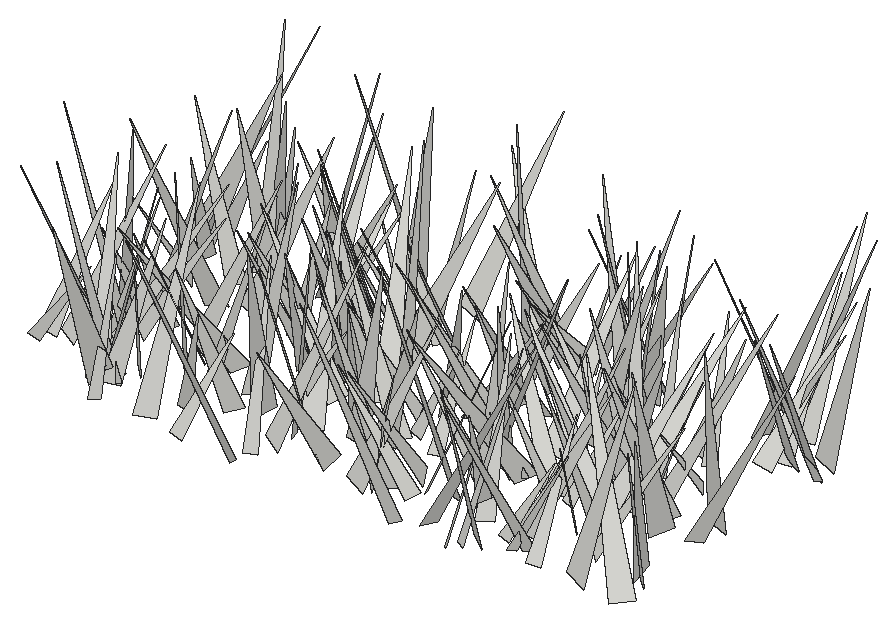
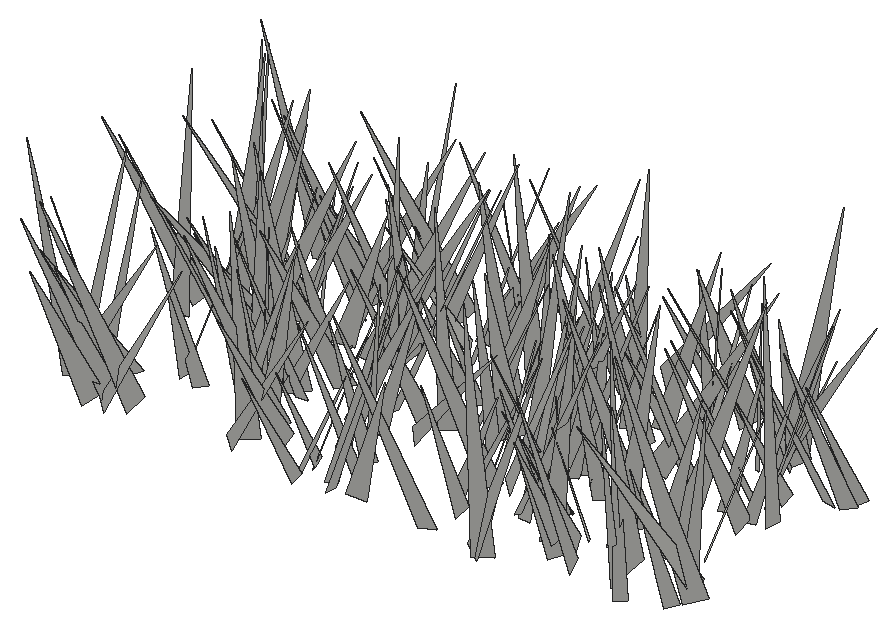
# SketchUp Ruby script. Lengths in inches.
U = 1.inch
M = Sketchup.active_model
def pt(a) = Geom::Point3d.new(a.map { |v| v * U })
def face(e, loops, mat)
  f = e.add_face(loops[0].map { |a| pt(a) })
  loops[1..].each { |l| e.add_face(l.map { |a| pt(a) }).erase! }
  f.material = f.back_material = mat if mat
  f
end
# faces: each face lists its corners as indices into pts; further lists are holes
def faces(e, pts, list, mat = nil) = list.each { |f| face(e, (f[0].is_a?(Array) ? f : [f]).map { |l| l.map { |i| pts[i] } }, mat) }
# xy, xz, yz: faces in a plane at the given z, y or x. An outline is a flat list of corners, or four numbers for a rectangle; further outlines are holes
def ring(l) = l.size == 4 ? [[l[0], l[1]], [l[2], l[1]], [l[2], l[3]], [l[0], l[3]]] : l.each_slice(2).to_a
def flat(e, list, mat, &to3) = list.each { |f| face(e, (f[0].is_a?(Array) ? f : [f]).map { |l| ring(l).map { |u, v| to3.(u, v) } }, mat) }
def xy(e, z, list, mat = nil) = flat(e, list, mat) { |x, y| [x, y, z] }
def xz(e, y, list, mat = nil) = flat(e, list, mat) { |x, z| [x, y, z] }
def yz(e, x, list, mat = nil) = flat(e, list, mat) { |y, z| [x, y, z] }
def lines(e, pts, list) = list.each { |a, b| e.add_line(pt(pts[a]), pt(pts[b])) }
# prism: a flat outline (further loops are holes) pulled along v
def prism(e, loops, v, mat = nil)
  f = face(e, loops, mat); d = Geom::Vector3d.new(v.map { |x| x * U })
  f.pushpull(f.normal.samedirection?(d) ? d.length : -d.length)
end
def box(e, o, s, mat = nil) = prism(e, [[o, [o[0] + s[0], o[1], o[2]], [o[0] + s[0], o[1] + s[1], o[2]], [o[0], o[1] + s[1], o[2]]]], [0, 0, s[2]], mat)
def at(x, y, z, deg = 0) = Geom::Transformation.translation(pt([x, y, z])) * Geom::Transformation.rotation(ORIGIN, Z_AXIS, deg.degrees)
def axes(o, x, y, z) = Geom::Transformation.new([*x, 0, *y, 0, *z, 0, *pt(o).to_a, 1])
def part(name) = M.definitions.add(name)
# library, detail: a bought-in or finely detailed component or shape, given as its bounding box
def library(name, o, s) = part(name).tap { |d| box(d.entities, o, s) }
def detail(e, o, s) = box(e.add_group.entities, o, s)
def put(e, d, t, mat = nil) = e.add_instance(d, t).tap { |i| i.material = mat if mat }
def group(e, t, mat = nil) = e.add_group.tap { |g| g.transformation = t; g.material = mat if mat }.entities
root = M.entities
c1 = part("fur_instance\#9")
p = [[0.8125,0,1.79],[0.67,-0.02,1.48],[0,-0.11,0],[0,0.11,0]]
faces(c1.entities,p,[[0,1,2,3]])
put(root,c1,axes([536.92,438.28,-21.66],[-3.51133,-6.12863,1.17286],[-5.90116,3.69891,1.66117],[2.0278,0.152,6.86513]))
put(root,c1,axes([505.61,439.67,-21.66],[5.60712,-6.07402,0.33398],[-5.83929,-5.5015,-2.02021],[-1.70529,-1.13347,8.01575]))
put(root,c1,axes([523.48,440.46,-21.66],[5.96418,-2.86813,1.57613],[-1.66285,-5.47776,-3.67572],[-2.81874,-2.83722,5.50334]))
put(root,c1,axes([518.46,436.68,-21.66],[-5.00631,-5.98003,0.73957],[-5.22244,3.82659,-4.41068],[-3.00563,3.31169,6.43193]))
put(root,c1,axes([531.37,436.94,-21.66],[-3.36679,-6.63148,1.92496],[-6.20382,1.96447,-4.08298],[-3.03226,3.34389,6.21619]))
put(root,c1,axes([540.28,439.35,-21.66],[-1.24481,-6.10899,0.55091],[-5.80958,0.99391,-2.10566],[-1.96776,0.93016,5.86818]))
put(root,c1,axes([513.62,436.97,-21.66],[-0.24087,4.17753,0.95098],[3.88217,0.61574,-1.72155],[1.81241,-0.76371,3.81393]))
put(root,c1,axes([535.84,436.43,-21.66],[2.63979,2.66437,0.28601],[2.37928,-2.51517,1.47039],[-1.23275,0.85099,3.4504]))
put(root,c1,axes([548.02,440.89,-21.66],[-3.37811,-5.89928,1.5704],[-5.1932,3.72048,2.80499],[3.2091,-0.18922,6.19235]))
put(root,c1,axes([544.89,438.19,-21.66],[-0.81294,-7.33898,4.00432],[-7.82592,2.08335,2.22952],[2.94113,3.51498,7.03923]))
put(root,c1,axes([511.96,440.06,-21.66],[0.90872,-5.0896,0.45336],[-4.90772,-0.74115,1.51668],[1.42262,0.69427,4.94262]))
put(root,c1,axes([529.14,442.67,-21.66],[-5.60645,-3.595,0.79099],[-2.74257,5.04084,3.47133],[2.4552,-2.57833,5.68385]))
put(root,c1,axes([547.64,441.39,-21.66],[7.1612,-0.61813,1.17268],[-0.1707,-6.81898,-2.55193],[-1.31459,-2.48182,6.71956]))
put(root,c1,axes([527.31,439.58,-21.66],[3.73633,3.15118,1.53756],[3.50493,-3.41917,-1.50964],[-0.09758,-2.15258,4.64878]))
put(root,c1,axes([530.17,440.2,-21.66],[-4.08347,2.98679,1.40676],[3.27171,3.36098,2.36101],[-0.44252,-2.71247,4.47451]))
put(root,c1,axes([506.64,437.51,-21.66],[-4.46885,1.59045,1.08144],[1.18804,4.43404,-1.61169],[1.51249,1.21632,4.46123]))
put(root,c1,axes([535.125,441.41,-21.66],[4.67947,-2.49587,0.44393],[-2.29207,-4.56374,-1.49753],[-1.08298,-1.12554,5.08765]))
put(root,c1,axes([526.33,439.14,-21.66],[1.93796,6.92662,2.2466],[6.80944,-0.90011,-3.09877],[2.58009,-2.82714,6.49087]))
put(root,c1,axes([533.09,438.17,-21.66],[7.82793,-0.68601,0.13891],[-0.69946,-7.6099,1.83483],[0.02566,1.8399,7.64072]))
put(root,c1,axes([548.9,437.92,-21.66],[-3.56857,7.17935,0.49748],[7.02506,3.35468,1.97986],[-1.56176,-1.31463,7.76903]))
put(root,c1,axes([514.4375,441.86,-21.66],[2.95346,-5.37759,1.21149],[-5.08452,-3.18852,-1.75785],[-2.12927,0.1548,5.87804]))
put(root,c1,axes([538,439.58,-21.66],[1.07989,-3.22676,1.49499],[-3.22529,-0.23045,1.83235],[1.49815,1.82977,2.86716]))
put(root,c1,axes([528.29,440.17,-21.66],[-0.67807,6.71445,3.30984],[6.96597,-0.65101,2.74773],[-2.74118,-3.31527,6.16389]))
put(root,c1,axes([536.34,437.25,-21.66],[4.01654,5.38759,0.39242],[5.219,-3.99648,1.45013],[-1.3936,0.56102,6.56169]))
put(root,c1,axes([516.14,442.76,-21.66],[7.64117,-3.1953,0.94942],[-2.87226,-7.51641,-2.18001],[-1.69158,-1.67105,7.9903]))
put(root,c1,axes([539.35,438.72,-21.66],[3.96425,-0.56902,0.64503],[-0.79665,-3.57598,1.74151],[-0.32433,1.82859,3.60641]))
put(root,c1,axes([522.51,440.26,-21.66],[-5.08452,-4.09315,0.88657],[-4.17476,4.84247,-1.58557],[-0.33349,1.78573,6.33184]))
put(root,c1,axes([506.54,442.16,-21.66],[-2.8265,-4.26887,1.57231],[-3.66111,3.23328,2.19698],[2.70032,-0.08465,4.62446]))
put(root,c1,axes([506.38,439.875,-21.66],[-3.06653,-6.21678,2.70439],[-6.51984,1.89062,-3.04678],[-1.85842,3.62531,6.22648]))
put(root,c1,axes([506.16,439.67,-21.66],[-3.15581,4.82371,2.67558],[4.59437,4.00448,-1.80054],[3.05265,-1.04019,5.47589]))
put(root,c1,axes([518.74,438.11,-21.66],[0.42359,6.38348,0.10104],[6.1795,-0.43539,1.60081],[-1.60398,0.00839,6.194]))
put(root,c1,axes([541.57,438.09,-21.66],[-3.94545,3.07895,0.18102],[2.74281,3.63702,-2.08047],[1.41057,1.53994,4.55172]))
put(root,c1,axes([510.56,437.71,-21.66],[-6.29891,4.40553,1.36932],[3.82289,6.28157,-2.62437],[2.58248,1.44677,7.22479]))
put(root,c1,axes([504.68,442.55,-21.66],[-4.29176,-1.39668,0.34406],[-1.22552,4.11722,1.42648],[0.75311,-1.25938,4.28195]))
put(root,c1,axes([505.99,441.15,-21.66],[-4.67528,-5.85921,0.505],[-5.43274,4.05599,-3.23694],[-2.25181,2.37953,6.76097]))
put(root,c1,axes([498.68,441.33,-21.66],[1.93678,-3.59499,0.72466],[-3.24209,-1.29543,2.2385],[1.71404,1.61186,3.41529]))
put(root,c1,axes([518.97,440.01,-21.66],[3.76818,7.24013,0.96766],[7.17608,-3.46602,-2.01138],[1.36373,-1.76699,7.91031]))
put(root,c1,axes([538.77,440.88,-21.66],[3.61026,-5.57217,1.81458],[-5.57053,-2.60139,3.09478],[1.81959,3.09184,5.87413]))
put(root,c1,axes([532.58,441.68,-21.66],[-5.1387,-6.17044,1.38685],[-6.22365,4.61615,-2.52214],[-1.12419,2.64967,7.62361]))
put(root,c1,axes([540.75,443.41,-21.66],[-2.708,-3.38854,1.07596],[-2.8715,2.88211,1.84961],[2.09627,-0.42942,3.92357]))
put(root,c1,axes([523.2,443.43,-21.66],[1.45469,-7.67033,1.86376],[-7.74266,-1.0178,1.85445],[1.53584,2.13396,7.5836]))
put(root,c1,axes([504.99,439.85,-21.66],[-6.13848,3.83375,0.83292],[3.60337,6.1212,-1.61832],[1.55148,0.95163,7.05405]))
put(root,c1,axes([543.63,441.62,-21.66],[3.84668,4.92623,0.09388],[4.62666,-3.57049,-2.21792],[1.69428,-1.43435,5.84342]))
put(root,c1,axes([510.96,441.5,-21.66],[-6.29577,-3.22015,2.48262],[-3.79064,6.30377,-1.43636],[1.47099,2.46225,6.92409]))
put(root,c1,axes([532.69,444.27,-21.66],[-6.28485,-0.79991,0.77187],[-0.56549,6.11624,1.73401],[0.95701,-1.63912,6.09364]))
put(root,c1,axes([534.32,446.5,-21.66],[4.16443,-6.48584,0.7003],[-5.50995,-3.94185,-3.74183],[-3.49241,-1.51483,6.7385]))
put(root,c1,axes([505.3,440.26,-21.66],[5.32876,3.34285,1.26399],[2.90072,-5.37113,1.97605],[-2.08763,1.0697,5.97207]))
put(root,c1,axes([508.51,445.92,-21.66],[-3.43446,-5.67079,0.15135],[-5.3482,3.29577,2.1239],[1.89143,-0.97791,6.28032]))
put(root,c1,axes([535.67,440.57,-21.66],[-5.09281,3.29268,0.78292],[3.01884,5.05892,-1.63872],[1.53013,0.9783,5.83893]))
put(root,c1,axes([511.47,446.3,-21.66],[2.28844,-6.77562,0.58153],[-5.77223,-2.2597,-3.61376],[-3.59563,-0.68473,6.17144]))
put(root,c1,axes([519.42,441.7,-21.66],[-5.36603,-1.88935,2.74168],[-2.67241,5.54565,-1.40882],[1.98613,2.35731,5.51173]))
put(root,c1,axes([524.52,444.48,-21.66],[2.49015,-6.48815,0.76577],[-6.33726,-2.19962,1.97082],[1.58797,1.39602,6.66429]))
put(root,c1,axes([538.21,442.54,-21.66],[4.07945,6.65627,1.20942],[6.56454,-3.55321,-2.58689],[1.63565,-2.3408,7.36585]))
put(root,c1,axes([517.45,443.27,-21.66],[1.13497,4.33314,1.68645],[4.04549,-0.06445,-2.557],[2.29221,-2.03177,3.67778]))
put(root,c1,axes([545.28,446.41,-21.66],[6.81384,-4.6319,0.82302],[-4.34734,-6.75311,-2.01405],[-1.7979,-1.22528,7.98915]))
put(root,c1,axes([498.96,442.43,-21.66],[-0.64371,5.67181,1.6895],[5.48083,1.21245,-1.9821],[2.23257,-1.34117,5.35305]))
put(root,c1,axes([521.33,445.53,-21.66],[5.7747,-1.11479,0.95698],[-0.77258,-5.60537,-1.86777],[-1.24967,-1.68603,5.57685]))
put(root,c1,axes([541.55,444.47,-21.66],[-0.61117,-4.98438,1.28841],[-4.9544,0.21679,-1.51148],[-1.3993,1.40945,4.78884]))
put(root,c1,axes([530.46,441.21,-21.66],[5.39727,3.08007,0.18691],[2.81936,-5.07536,2.22356],[-1.25418,1.84558,5.80286]))
put(root,c1,axes([503.61,442.96,-21.66],[4.07618,6.66518,0.05677],[6.29765,-3.82934,-2.59208],[2.18344,-1.39809,7.37028]))
put(root,c1,axes([532.86,446.38,-21.66],[-0.95701,-7.3765,1.52863],[-7.35851,1.24531,1.40248],[1.61303,1.30453,7.30491]))
put(root,c1,axes([500.32,442.69,-21.66],[3.27574,7.01328,0.4286],[6.91428,-3.13335,-1.57325],[1.25002,-1.04703,7.57902]))
put(root,c1,axes([533.96,446.21,-21.66],[-0.88156,-7.55851,1.51866],[-6.98391,0.13553,-3.37952],[-3.26533,1.75074,6.81814]))
put(root,c1,axes([543.74,443.61,-21.66],[-5.8174,-1.77979,0.63377],[-1.88895,5.44209,-2.05595],[-0.03436,2.15114,5.72563]))
put(root,c1,axes([544.56,447.98,-21.66],[4.80853,-5.64104,1.01196],[-5.19564,-4.8483,-2.3381],[-2.41883,-0.80002,7.03396]))
put(root,c1,axes([520.33,447.39,-21.66],[7.53052,-1.13144,2.64431],[-0.30654,-7.68469,-2.41514],[-2.85982,-2.15562,7.22191]))
put(root,c1,axes([503.62,444.63,-21.66],[-7.70081,-2.50661,0.76749],[-2.60656,7.57519,-1.4131],[0.27927,1.58364,7.97425]))
put(root,c1,axes([539.65,447.16,-21.66],[-5.8383,-2.13052,1.19785],[-1.77007,5.82456,1.73238],[1.68547,-1.263,5.96857]))
put(root,c1,axes([525.01,445.45,-21.66],[-3.75455,5.21199,1.89568],[5.51913,3.28609,1.89629],[-0.5456,-2.62523,6.13723]))
put(root,c1,axes([536.98,445.66,-21.66],[-0.30638,-3.92044,1.36874],[-3.76361,-0.31774,-1.75256],[-1.75458,1.36615,3.52026]))
put(root,c1,axes([541.44,445.42,-21.66],[-6.06762,4.08752,0.30456],[4.00596,5.79855,1.98636],[-0.86766,-1.81261,7.04117]))
put(root,c1,axes([514.07,444.28,-21.66],[6.87844,-2.02965,2.77665],[-2.6588,-7.07628,1.41394],[-2.18175,2.22463,7.03088]))
put(root,c1,axes([519.76,442.93,-21.66],[-5.97227,4.9002,0.90124],[4.6479,5.98621,-1.7477],[1.79477,0.80344,7.52499]))
put(root,c1,axes([501.39,447.05,-21.66],[7.9282,0.66664,2.15118],[1.11346,-8.00329,-1.62351],[-1.9576,-1.85234,7.78877]))
put(root,c1,axes([504.76,447.6,-21.66],[3.23703,-3.40023,0.62778],[-3.13183,-3.24768,-1.44163],[-1.46538,-0.57015,4.46784]))
put(root,c1,axes([502.75,447.79,-21.66],[3.29812,-3.00828,0.87507],[-2.53709,-3.30998,-1.81667],[-1.83812,-0.82908,4.07763]))
put(root,c1,axes([542.24,443.01,-21.66],[1.49345,8.09623,0.02611],[7.76227,-1.42429,-2.34489],[2.30146,-0.44999,7.89182]))
put(root,c1,axes([532.88,444.05,-21.66],[7.43701,2.08557,1.03262],[1.85087,-7.39668,1.60887],[-1.41074,1.29018,7.55449]))
put(root,c1,axes([532.56,444.4,-21.66],[-6.83852,1.49302,2.47832],[0.97247,7.17644,-1.63995],[2.72497,1.18576,6.80477]))
put(root,c1,axes([517.67,449.05,-21.66],[-0.91329,-6.82842,0.06821],[-6.63421,0.90353,1.6239],[1.61843,-0.14959,6.69511]))
put(root,c1,axes([502.67,444.01,-21.66],[4.59265,0.40937,1.72839],[-0.43371,-4.3881,2.19176],[-1.72245,2.19644,4.05662]))
put(root,c1,axes([541.54,448.83,-21.66],[1.64942,-7.33453,1.1804],[-6.83961,-1.97125,-2.69132],[-2.89974,0.47759,7.01946]))
put(root,c1,axes([503.59,445.96,-21.66],[3.2036,5.15972,0.63397],[4.7617,-2.61371,-2.78969],[2.08586,-1.95793,5.39475]))
put(root,c1,axes([518.72,446.99,-21.66],[-6.43604,2.78332,0.65453],[2.85741,6.20344,1.71766],[-0.1023,-1.83529,6.79846]))
put(root,c1,axes([538.4,445.58,-21.66],[0.79551,4.29487,0.6755],[4.10301,-0.51451,-1.56067],[1.4379,-0.90797,4.07959]))
put(root,c1,axes([514.33,449.23,-21.66],[6.011,-2.52803,0.45147],[-2.2406,-5.7244,-2.22212],[-1.25478,-1.8887,6.13068]))
put(root,c1,axes([523.875,448.8,-21.66],[-4.91943,-1.92287,0.32626],[-1.70701,4.67316,1.80343],[0.9434,-1.57124,4.96446]))
put(root,c1,axes([525.36,446.48,-21.66],[0.91676,-3.52562,1.5814],[-3.59518,-0.18259,1.67709],[1.41617,1.81877,3.23385]))
put(root,c1,axes([515.92,449.16,-21.66],[4.34994,-4.04005,0.73934],[-3.73736,-4.34022,-1.72779],[-1.70317,-0.79441,5.67968]))
put(root,c1,axes([536.98,445.85,-21.66],[-3.95209,5.35159,0.47213],[5.26841,3.74586,1.6413],[-1.05182,-1.34553,6.44707]))
put(root,c1,axes([510.95,443.93,-21.66],[5.49101,0.89671,2.25711],[-0.37206,-5.20349,2.97239],[-2.40004,2.85822,4.70322]))
put(root,c1,axes([529.14,450.52,-21.66],[-7.53778,-2.79862,0.78068],[-2.32716,7.11502,3.03655],[1.73954,-2.60846,7.44512]))
put(root,c1,axes([514.14,444.78,-21.66],[-6.72177,-1.11045,3.37602],[-2.29516,6.87097,-2.30972],[2.71346,3.06096,6.4094]))
put(root,c1,axes([547.55,449.13,-21.66],[-1.05079,-7.8114,1.55453],[-7.7743,1.34665,1.51176],[1.73053,1.30661,7.73542]))
put(root,c1,axes([514.99,450.18,-21.66],[-6.3203,-1.31951,1.76492],[-0.3807,5.93404,3.07318],[2.17051,-2.80147,5.67828]))
put(root,c1,axes([527.96,445.26,-21.66],[-3.50119,3.09472,0.56001],[2.74674,3.41714,-1.71109],[1.53177,0.94611,4.34831]))
put(root,c1,axes([541.5,449.23,-21.66],[3.93699,-6.31061,2.13001],[-6.14082,-4.39732,-1.67764],[-2.57895,0.83692,7.24632]))
put(root,c1,axes([507.51,446.85,-21.66],[3.41975,6.53108,1.33927],[6.45057,-2.86091,-2.51965],[1.68487,-2.30293,6.92828]))
put(root,c1,axes([513.57,450.0625,-21.66],[-5.24067,-3.21189,0.67738],[-2.84495,5.08085,2.08111],[1.63749,-1.45206,5.78359]))
put(root,c1,axes([537.84,446.4,-21.66],[4.12915,-1.39251,2.24683],[-2.1688,-4.1671,1.40312],[-1.51116,2.17563,4.12556]))
put(root,c1,axes([524.98,450.3125,-21.66],[6.92696,-1.79403,0.01467],[-1.72828,-6.68834,-1.86567],[-0.48147,-1.80253,6.90801]))
put(root,c1,axes([547.625,446.75,-21.66],[6.83257,-2.01041,0.78824],[-2.1593,-6.33413,2.56189],[0.022,2.68032,6.64549]))
put(root,c1,axes([539.23,449.9375,-21.66],[3.81645,-5.44593,0.15233],[-5.28758,-3.65777,1.70554],[1.31259,1.09964,6.42764]))
put(root,c1,axes([505.22,451.65,-21.66],[0.76231,-8.24421,0.75454],[-8.09051,-0.90251,-1.68715],[-1.75496,0.57958,8.10565]))
put(root,c1,axes([542.89,447.95,-21.66],[4.06306,2.1594,0.43468],[1.91332,-3.91175,1.54848],[-1.0914,1.18135,4.33286]))
put(root,c1,axes([543.72,452.49,-21.66],[-3.33896,-2.6162,0.26799],[-2.1089,2.92233,2.25332],[1.57125,-1.6372,3.59384]))
put(root,c1,axes([518.61,450.53,-21.66],[-0.87207,-5.64239,2.10409],[-5.67136,0.05471,-2.20385],[-2.02471,2.277,5.26688]))
put(root,c1,axes([526.8,450.24,-21.66],[4.24231,-3.44067,0.07958],[-3.18347,-3.87509,2.16585],[1.3077,1.72835,5.01442]))
put(root,c1,axes([516.79,449.17,-21.66],[1.83922,3.08635,0.93557],[2.6886,-2.06216,1.51739],[-1.78108,0.07419,3.25666]))
put(root,c1,axes([502.75,448.33,-21.66],[7.28027,0.47928,1.68125],[-0.05604,-7.13268,2.27604],[-1.74733,2.22571,6.93193]))
put(root,c1,axes([501.88,453.28,-21.66],[-3.67716,-3.23058,0.06887],[-2.92053,3.36739,2.02339],[1.38271,-1.47883,4.45691]))
put(root,c1,axes([515.23,453,-21.66],[2.94915,-5.28887,0.70098],[-5.06545,-3.02722,-1.5291],[-1.67475,-0.15728,5.85931]))
put(root,c1,axes([535.37,452.36,-21.66],[3.43501,-7.39782,1.03394],[-7.28345,-3.06455,2.27067],[1.65774,1.86463,7.83397]))
put(root,c1,axes([538.72,453.67,-21.66],[3.46816,-3.92613,0.03464],[-3.68547,-3.27126,-1.77763],[-1.35388,-1.15247,4.92774]))
put(root,c1,axes([511.85,451.26,-21.66],[0.68635,-5.64905,2.27441],[-5.90756,-0.06201,1.6287],[1.47832,2.3749,5.45254]))
put(root,c1,axes([540.49,449.05,-21.66],[5.57667,1.59527,0.3002],[1.43066,-5.3377,1.78788],[-0.76695,1.64269,5.51794]))
put(root,c1,axes([530.14,453.46,-21.66],[-0.06223,-5.95217,0.13196],[-5.73579,0.02457,-1.59678],[-1.59576,0.14382,5.73432]))
put(root,c1,axes([540.73,449.33,-21.66],[-0.59735,8.07244,1.41711],[8.08686,0.34954,1.4177],[-1.33238,-1.49761,7.96939]))
put(root,c1,axes([521.26,448.54,-21.66],[-6.0602,5.67803,0.65626],[5.53411,6.06799,-1.39639],[1.4298,0.57987,8.18634]))
put(root,c1,axes([541.33,447.48,-21.66],[-3.48939,6.7058,0.49493],[5.71017,3.24965,-3.77124],[3.55058,1.36403,6.55144]))
put(root,c1,axes([528.06,453.49,-21.66],[2.83348,-4.00549,0.52306],[-3.76222,-2.8494,-1.43972],[-1.47079,-0.42795,4.69039]))
put(root,c1,axes([542.59,450.06,-21.66],[4.68977,6.59581,0.10077],[6.41242,-4.52929,-1.96857],[1.54784,-1.22048,7.85006]))
put(root,c1,axes([518.68,454.1,-21.66],[-3.83157,-3.11067,0.41222],[-2.87249,3.73899,1.51524],[1.26294,-0.9332,4.69694]))
put(root,c1,axes([535.94,452.9,-21.66],[-4.58905,2.11277,0.48874],[2.15665,4.32669,1.54618],[-0.22698,-1.60562,4.80963]))
put(root,c1,axes([521.66,449.83,-21.66],[-7.99125,0.08509,2.25297],[-0.74491,7.73167,-2.93422],[2.12796,3.02611,7.43355]))
put(root,c1,axes([507.37,452.31,-21.66],[1.82991,-7.19945,3.13467],[-7.38413,-0.48301,3.20126],[2.67073,3.59742,6.70317]))
put(root,c1,axes([533.54,449.92,-21.66],[-2.62249,6.7547,0.84995],[6.3246,2.75431,-2.37468],[2.5195,0.11678,6.84575]))
put(root,c1,axes([526.19,452.23,-21.66],[-4.35257,-4.39527,0.35538],[-3.69396,3.36161,-3.66659],[-2.40819,2.78761,4.98191]))
put(root,c1,axes([513.97,456.35,-21.66],[-3.49524,-7.20934,0.56433],[-6.86604,3.50524,2.25399],[2.26947,-0.49846,7.68835]))
put(root,c1,axes([507.14,455.24,-21.66],[6.25935,-4.83068,2.00086],[-4.50057,-6.56633,-1.77386],[-2.66155,-0.25726,7.70509]))
put(root,c1,axes([517.51,453.64,-21.66],[-4.9951,-5.23204,0.99068],[-5.30492,4.77148,-1.54841],[-0.46216,1.77916,7.06595]))
put(root,c1,axes([519.05,455.41,-21.66],[-4.78281,-0.5343,0.54387],[-0.29464,4.48183,1.81189],[0.70318,-1.75621,4.45846]))
put(root,c1,axes([538.27,452.18,-21.66],[-6.12572,-2.31991,2.2614],[-2.97153,5.95041,-1.94497],[1.2907,2.68904,6.25488]))
put(root,c1,axes([540.75,451.73,-21.66],[-5.40299,1.91129,1.15946],[1.49374,5.34299,-1.84687],[1.66317,1.41036,5.42535]))
put(root,c1,axes([500.91,456.07,-21.66],[4.81338,-2.70132,0.36004],[-2.51999,-4.69011,-1.49931],[-1.0375,-1.14068,5.31205]))
put(root,c1,axes([534.7,452.91,-21.66],[1.84734,5.85191,0.92453],[5.8229,-1.61485,-1.41361],[1.09242,-1.28828,5.97153]))
put(root,c1,axes([528.67,456.32,-21.66],[3.08843,-3.08617,0.55459],[-2.71507,-3.02147,-1.69397],[-1.56857,-0.84658,4.0241]))
put(root,c1,axes([510.92,457.39,-21.66],[6.38764,-4.10189,0.26345],[-3.90919,-6.21298,-1.95294],[-1.27011,-1.50671,7.33577]))
put(root,c1,axes([512.29,453.85,-21.66],[3.25743,4.86298,0.41292],[4.6269,-2.91916,-2.12138],[1.55271,-1.50328,5.4552]))
put(root,c1,axes([514.6,455.61,-21.66],[-6.87538,0.87455,0.95023],[1.06547,6.75006,1.49673],[0.72976,-1.61573,6.76724]))
put(root,c1,axes([504.45,454.57,-21.66],[0.94645,-5.69848,3.07489],[-6.04954,-1.88624,-1.63358],[-2.30884,2.60631,5.54074]))
put(root,c1,axes([515.64,457.98,-21.66],[-3.26721,-5.06008,0.08616],[-4.54982,2.98181,2.58736],[2.21606,-1.33826,5.43917]))
put(root,c1,axes([518.34,454.16,-21.66],[2.77972,-6.83526,2.99642],[-7.05556,-1.36449,3.4327],[2.43278,3.85274,6.53179]))
put(root,c1,axes([548.21,458.24,-21.66],[-2.24137,-6.8028,0.2078],[-6.58087,2.22202,1.76064],[1.73594,-0.35988,6.94277]))
put(root,c1,axes([509.16,455.8,-21.66],[3.22787,2.03353,0.24614],[1.96333,-2.94045,-1.45397],[0.58408,-1.35405,3.52709]))
put(root,c1,axes([540.63,455.62,-21.66],[1.73127,-4.9492,1.56465],[-4.93445,-1.0575,2.11492],[1.61056,2.08017,4.79781]))
put(root,c1,axes([546.29,458.33,-21.66],[-1.98153,-6.18192,0.39554],[-6.00617,2.01899,1.46585],[1.5161,-0.08133,6.32408]))
put(root,c1,axes([512.44,453.98,-21.66],[-0.90144,4.87523,0.09791],[4.65666,0.89022,-1.45364],[1.44671,0.1723,4.73998]))
put(root,c1,axes([538.56,454.34,-21.66],[6.05789,3.57549,2.196],[3.19122,-6.43003,1.66595],[-2.72445,0.41853,6.83424]))
put(root,c1,axes([536.97,455.9,-21.66],[-4.91979,-5.33902,1.78444],[-5.59743,4.38767,-2.30455],[-0.5985,2.85253,6.88466]))
put(root,c1,axes([526.5,460.17,-21.66],[-6.90134,-2.30385,2.57209],[-0.73953,6.60101,3.92832],[3.37291,-3.26662,6.12409]))
put(root,c1,axes([528.46,459.57,-21.66],[-4.47086,-3.62986,0.22446],[-3.11938,4.01034,2.72058],[1.8697,-1.98902,5.07572]))
put(root,c1,axes([519.24,456.55,-21.66],[-1.9475,3.70978,1.3462],[3.85912,1.47603,1.51527],[-0.82582,-1.85103,3.9063]))
put(root,c1,axes([526.14,456.74,-21.66],[2.61538,-3.98544,0.72253],[-3.93735,-2.29982,1.56655],[0.95028,1.43982,4.50221]))
put(root,c1,axes([536.58,454.35,-21.66],[4.8815,3.3845,2.02519],[2.72156,-5.22275,2.16824],[-2.85471,0.80828,5.53015]))
put(root,c1,axes([534.08,459,-21.66],[2.99312,-6.69994,0.30324],[-6.59145,-2.87731,1.48788],[1.23852,0.87852,7.18569]))
put(root,c1,axes([542.27,454.95,-21.66],[-4.53148,2.02632,0.31118],[1.79338,4.28391,-1.78018],[0.99329,1.50971,4.63371]))
put(root,c1,axes([516.61,456.76,-21.66],[0.00954,3.59248,1.3323],[3.47361,-0.5704,1.51319],[-1.6171,-1.20405,3.25826]))
put(root,c1,axes([499.05,457.74,-21.66],[3.50419,-7.42751,1.71848],[-7.22357,-2.63012,3.36199],[2.43745,2.88357,7.49295]))
put(root,c1,axes([528.83,460.54,-21.66],[-4.31312,-2.31019,0.44376],[-1.59331,3.55068,2.99849],[1.73068,-2.4885,3.8664]))
put(root,c1,axes([533.3125,456.69,-21.66],[6.82569,-2.14516,0.01525],[-2.06759,-6.56497,1.95405],[0.57187,1.86856,6.88284]))
put(root,c1,axes([535.32,455.44,-21.66],[0.70112,8.01126,1.73468],[7.49163,-1.33281,3.12731],[-3.32639,-1.31314,7.4089]))
put(root,c1,axes([502.8125,460.64,-21.66],[-1.84089,-7.99139,1.4242],[-7.16502,2.28604,3.56596],[3.81486,0.4373,7.3848]))
put(root,c1,axes([548.77,457.75,-21.66],[-3.53185,-5.19128,1.06072],[-4.89285,2.7062,-3.04713],[-2.03336,2.50511,5.48984]))
put(root,c1,axes([509.48,458.82,-21.66],[2.07826,-5.21506,0.82935],[-4.82149,-1.51054,2.58366],[2.15357,1.65083,4.98405]))
put(root,c1,axes([525.89,458.24,-21.66],[1.52671,4.77623,1.67607],[4.63081,-0.61106,-2.47682],[2.04382,-2.18327,4.35989]))
put(root,c1,axes([525.93,460.92,-21.66],[-7.13222,-2.21187,1.52983],[-1.72076,7.08542,2.22194],[2.06682,-1.73369,7.12909]))
put(root,c1,axes([525.84,457.25,-21.66],[-7.59721,-1.99805,2.32928],[-2.54922,7.5713,-1.81993],[1.70857,2.41215,7.64184]))
put(root,c1,axes([503.9375,459.64,-21.66],[-0.90647,-5.11686,1.80724],[-5.12934,1.40604,1.40817],[1.7715,1.45288,5.00209]))
put(root,c1,axes([499.84,459.15,-21.66],[2.80159,-3.67069,0.58517],[-3.61323,-2.51742,1.50747],[0.87232,1.36159,4.36468]))
put(root,c1,axes([547.84,459.6,-21.66],[2.12208,6.92928,3.4126],[7.54208,-1.09525,-2.46604],[1.66665,-3.86645,6.81445]))
put(root,c1,axes([543.3125,460.1875,-21.66],[5.8756,3.65861,0.2575],[3.32747,-5.11292,-3.2803],[1.54262,-2.90637,6.0949]))
put(root,c1,axes([509.48,456.55,-21.66],[4.83042,2.64277,1.00625],[2.0268,-4.62442,2.4159],[-1.97202,1.72053,4.9478]))
put(root,c1,axes([504.77,456.82,-21.66],[-7.79963,1.89477,1.60693],[1.33324,7.65978,-2.56065],[2.09639,2.17814,7.60707]))
put(root,c1,axes([517.64,458,-21.66],[5.12063,-0.00436,1.95562],[-0.62511,-5.19742,1.62522],[-1.85303,1.74129,4.85588]))
put(root,c1,axes([534.72,460.18,-21.66],[-3.87014,-4.65436,0.40491],[-4.4497,3.51193,-2.16136],[-1.42379,1.67578,5.65416]))
put(root,c1,axes([544.94,456.96,-21.66],[-2.23637,5.81255,0.47787],[5.16217,2.21098,-2.73477],[2.71405,0.58421,5.59536]))
put(root,c1,axes([513.07,461.67,-21.66],[1.49707,-8.01218,1.60299],[-8.01526,-1.12338,1.87068],[1.58751,1.88383,7.93327]))
put(root,c1,axes([528.8,458.63,-21.66],[3.99187,0.97882,1.10255],[0.50795,-3.90054,1.62373],[-1.38409,1.39155,3.77579]))
put(root,c1,axes([499.76,456.43,-21.66],[7.75154,3.11882,0.30174],[2.75499,-7.16733,3.30818],[-1.4927,2.96765,7.67264]))
put(root,c1,axes([509.52,457.92,-21.66],[-3.94963,4.34285,0.40783],[4.0226,3.83915,-1.92507],[1.68683,1.01332,5.54563]))
put(root,c1,axes([513.98,461.58,-21.66],[-4.11377,-6.51171,1.45116],[-6.65439,3.88319,-1.43913],[-0.47668,1.98739,7.56666]))
put(root,c1,axes([531.94,457.78,-21.66],[6.07778,0.82962,2.17123],[-0.33597,-5.70106,3.1188],[-2.29992,3.02515,5.28212]))
put(root,c1,axes([544.07,461.33,-21.66],[-4.22462,-4.77942,0.40733],[-4.62488,3.91455,-2.0354],[-1.27248,1.63999,6.04544]))
put(root,c1,axes([507.85,459.02,-21.66],[6.46332,2.41268,1.62775],[2.03661,-6.58136,1.66821],[-2.07914,1.05343,6.69422]))
put(root,c1,axes([545.66,458.05,-21.66],[-4.8564,4.18897,0.42907],[3.70643,4.56321,-2.59917],[1.99849,1.71635,5.86314]))
put(root,c1,axes([542.36,460.04,-21.66],[8.0865,0.10169,1.15451],[-0.2162,-7.86244,2.20681],[-1.13864,2.21504,7.78021]))
put(root,c1,axes([524.1,460.63,-21.66],[-2.5947,5.83184,0.30944],[5.66182,2.42897,1.69778],[-1.43174,-0.96349,6.15308]))
put(root,c1,axes([518.09,460.97,-21.66],[1.6055,7.88479,1.47704],[7.72527,-1.11383,-2.45126],[2.16141,-1.87581,7.66412]))
put(root,c1,axes([528.51,461.08,-21.66],[4.2696,-0.12633,0.87704],[-0.45536,-4.01534,1.6384],[-0.76014,1.6958,3.94476]))
put(root,c1,axes([544.22,460.2,-21.66],[7.47336,0.82298,1.26079],[0.38429,-7.21504,2.43175],[-1.45575,2.3203,7.11442]))
put(root,c1,axes([544.95,461.09,-21.66],[-6.41092,4.00729,0.82453],[3.32918,6.00061,-3.27831],[2.37798,2.40258,6.81256]))
